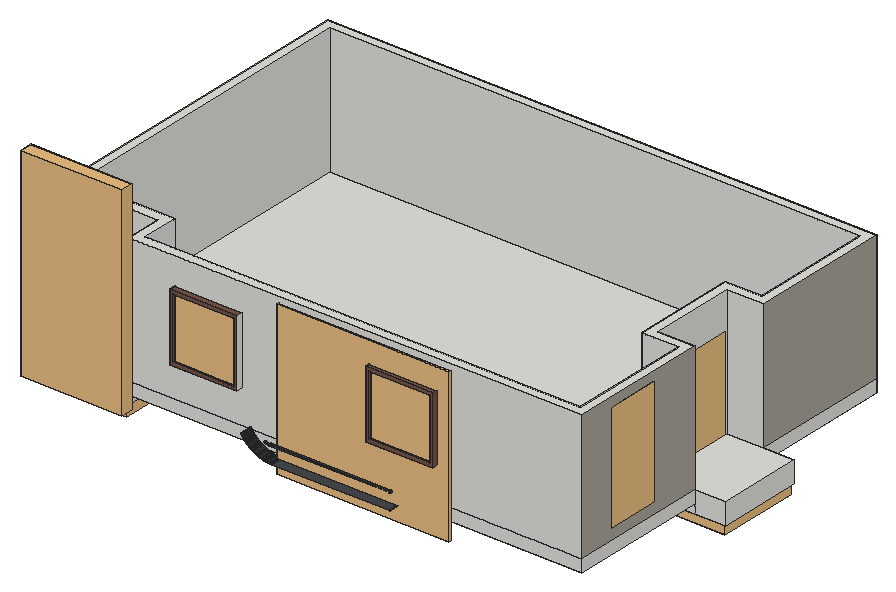
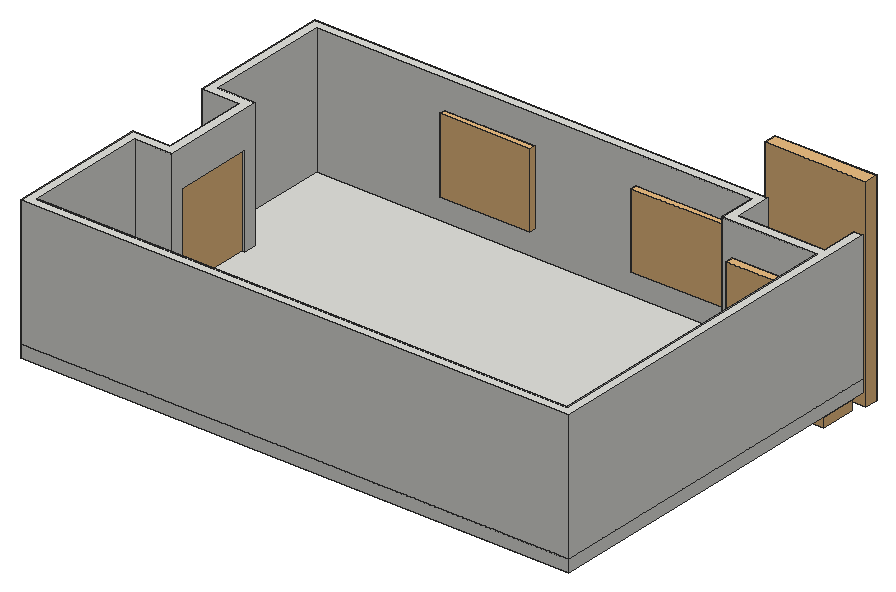
# SketchUp Ruby script. Lengths in inches.
U = 1.inch
M = Sketchup.active_model
def pt(a) = Geom::Point3d.new(a.map { |v| v * U })
def face(e, loops, mat)
  f = e.add_face(loops[0].map { |a| pt(a) })
  loops[1..].each { |l| e.add_face(l.map { |a| pt(a) }).erase! }
  f.material = f.back_material = mat if mat
  f
end
# faces: each face lists its corners as indices into pts; further lists are holes
def faces(e, pts, list, mat = nil) = list.each { |f| face(e, (f[0].is_a?(Array) ? f : [f]).map { |l| l.map { |i| pts[i] } }, mat) }
# xy, xz, yz: faces in a plane at the given z, y or x. An outline is a flat list of corners, or four numbers for a rectangle; further outlines are holes
def ring(l) = l.size == 4 ? [[l[0], l[1]], [l[2], l[1]], [l[2], l[3]], [l[0], l[3]]] : l.each_slice(2).to_a
def flat(e, list, mat, &to3) = list.each { |f| face(e, (f[0].is_a?(Array) ? f : [f]).map { |l| ring(l).map { |u, v| to3.(u, v) } }, mat) }
def xy(e, z, list, mat = nil) = flat(e, list, mat) { |x, y| [x, y, z] }
def xz(e, y, list, mat = nil) = flat(e, list, mat) { |x, z| [x, y, z] }
def yz(e, x, list, mat = nil) = flat(e, list, mat) { |y, z| [x, y, z] }
def lines(e, pts, list) = list.each { |a, b| e.add_line(pt(pts[a]), pt(pts[b])) }
# prism: a flat outline (further loops are holes) pulled along v
def prism(e, loops, v, mat = nil)
  f = face(e, loops, mat); d = Geom::Vector3d.new(v.map { |x| x * U })
  f.pushpull(f.normal.samedirection?(d) ? d.length : -d.length)
end
def box(e, o, s, mat = nil) = prism(e, [[o, [o[0] + s[0], o[1], o[2]], [o[0] + s[0], o[1] + s[1], o[2]], [o[0], o[1] + s[1], o[2]]]], [0, 0, s[2]], mat)
def at(x, y, z, deg = 0) = Geom::Transformation.translation(pt([x, y, z])) * Geom::Transformation.rotation(ORIGIN, Z_AXIS, deg.degrees)
def axes(o, x, y, z) = Geom::Transformation.new([*x, 0, *y, 0, *z, 0, *pt(o).to_a, 1])
def part(name) = M.definitions.add(name)
# library, detail: a bought-in or finely detailed component or shape, given as its bounding box
def library(name, o, s) = part(name).tap { |d| box(d.entities, o, s) }
def detail(e, o, s) = box(e.add_group.entities, o, s)
def put(e, d, t, mat = nil) = e.add_instance(d, t).tap { |i| i.material = mat if mat }
def group(e, t, mat = nil) = e.add_group.tap { |g| g.transformation = t; g.material = mat if mat }.entities
root = M.entities
M.materials.add("1111 AP 9939 Brown seed-N").color = [120, 84, 73]
M.materials.add("1432 AP 8245 TAR ROAD").color = [71, 72, 75]
M.materials.add("Generic").color = [172, 166, 153]
M.materials.add("Outer Light").color = [251, 217, 152]
M.materials.add("[Granite Dark Gray]").color = [69, 68, 68]
M.materials.add("[Wood Cherry Original]").color = [152, 86, 42]
M.materials.add("[Wood Veneer 01]").color = [120, 70, 37]
c1 = library("Group\#45",[0,-2,0],[63,2,36])
c2 = library("Group\#3",[-12,-12.5,-24],[99,12.5,198])
c3 = library("Double-hung window 69 in. x 58 in. triple row with mullions",[0,0,-3.59],[62,58,4.59])
c4 = library("Glass Door",[0,0,0],[72,3.54,96])
c5 = library("RIDEAUX \#16",[0,0,0],[103.86,7.74,93.57])
c6 = library("Curtain",[0,0,0],[121.12,7.86,100.24])
c7 = library("SLIDING+GLASS+DOOR",[0,-0.75,0],[72,5.75,80])
c8 = library("Group\#19",[0,0,0],[0.5,51,105])
c9 = library("Group\#46",[0,-2,0],[168,2,149.16])
c10 = library("Group\#56",[0,0,-17.09],[62,80,17.09])
c11 = library("Group\#32",[0,0,-17.09],[62,80,17.09])
xy(root,428.79,[[278.72,95.37,279,107.37],[279,95.37,393,107.37],[393,95.37,393.24,107.37],[393.24,95.37,393.47,107.37]],"1432 AP 8245 TAR ROAD")
xy(root,428.8,[[278.15,95.37,278.43,107.37]],"1432 AP 8245 TAR ROAD")
xy(root,444.29,[[278.68,95.37,278.84,96.87],[278.84,95.37,279,96.87],[279,95.37,393,96.87],[393,95.37,393.4375,96.87]],"1432 AP 8245 TAR ROAD")
xy(root,444.29,[[278.68,95.37,278.84,96.87],[278.84,95.37,279,96.87],[279,95.37,393,96.87],[393,95.37,393.4375,96.87]],"Outer Light")
xy(root,444.3,[[278.36,95.37,278.52,96.87]],"1432 AP 8245 TAR ROAD")
xy(root,444.3,[[278.36,95.37,278.52,96.87]],"Outer Light")
xy(root,444.31,[[278.03,95.37,278.2,96.87]],"1432 AP 8245 TAR ROAD")
xy(root,444.31,[[278.03,95.37,278.2,96.87]],"Outer Light")
xy(root,445.79,[[278.7,95.37,278.85,96.87],[278.85,95.37,279,96.87],[279,95.37,393,96.87],[393,95.37,393.46,96.87]],"1432 AP 8245 TAR ROAD")
xy(root,445.79,[[278.7,95.37,278.85,96.87],[278.85,95.37,279,96.87],[279,95.37,393,96.87],[393,95.37,393.46,96.87]],"Outer Light")
xy(root,445.8,[[278.4,95.37,278.55,96.87]],"1432 AP 8245 TAR ROAD")
xy(root,445.8,[[278.4,95.37,278.55,96.87]],"Outer Light")
p = [[394.18,107.37,428.75],[394.41,107.37,428.74],[394.41,95.37,428.74],[394.18,95.37,428.75],[394.65,107.37,428.72],[394.65,95.37,428.72],
  [394.88,107.37,428.69],[394.88,95.37,428.69],[276.74,107.37,428.86],[277.02,107.37,428.85],[277.02,95.37,428.85],[276.74,95.37,428.86],
  [277.3,107.37,428.83],[277.3,95.37,428.83],[277.59,107.37,428.82],[277.59,95.37,428.82],[277.87,107.37,428.81],[277.87,95.37,428.81],
  [278.15,107.37,428.8],[278.15,95.37,428.8],[278.43,107.37,428.8],[278.72,107.37,428.79],[278.72,95.37,428.79],[278.43,95.37,428.8],
  [393.47,107.37,428.79],[393.71,107.37,428.78],[393.71,95.37,428.78],[393.47,95.37,428.79],[393.94,107.37,428.77],[393.94,95.37,428.77],
  [275.61,107.37,428.95],[275.89,107.37,428.93],[275.89,95.37,428.93],[275.61,95.37,428.95],[276.18,107.37,428.9],[276.18,95.37,428.9],
  [276.46,107.37,428.88],[276.46,95.37,428.88],[274.49,107.37,429.08],[274.77,107.37,429.04],[274.77,95.37,429.04],[274.49,95.37,429.08],
  [275.05,107.37,429.01],[275.05,95.37,429.01],[275.33,107.37,428.98],[275.33,95.37,428.98],[273.93,107.37,429.15],[274.21,107.37,429.11],
  [274.21,95.37,429.11],[273.93,95.37,429.15],[273.09,107.37,429.28],[273.37,107.37,429.24],[273.37,95.37,429.24],[273.09,95.37,429.28],
  [273.65,107.37,429.19],[273.65,95.37,429.19],[272.53,107.37,429.38],[272.8125,107.37,429.33],[272.8125,95.37,429.33],[272.53,95.37,429.38],
  [271.98,107.37,429.48],[272.25,107.37,429.43],[272.25,95.37,429.43],[271.98,95.37,429.48],[271.42,107.37,429.6],[271.7,107.37,429.54],
  [271.7,95.37,429.54],[271.42,95.37,429.6],[271.15,107.37,429.66],[271.15,95.37,429.66],[270.6,107.37,429.79],[270.87,107.37,429.72],
  [270.87,95.37,429.72],[270.6,95.37,429.79],[270.32,107.37,429.85],[270.32,95.37,429.85],[269.77,107.37,429.99],[270.05,107.37,429.92],
  [270.05,95.37,429.92],[269.77,95.37,429.99],[269.5,107.37,430.07],[269.5,95.37,430.07],[268.96,107.37,430.22],[269.23,107.37,430.14],
  [269.23,95.37,430.14],[268.96,95.37,430.22],[268.69,107.37,430.3],[268.69,95.37,430.3],[268.41,107.37,430.38],[268.41,95.37,430.38],
  [268.14,107.37,430.47],[268.14,95.37,430.47],[267.875,107.37,430.55],[267.875,95.37,430.55],[267.34,107.37,430.73],[267.61,107.37,430.64],
  [267.61,95.37,430.64],[267.34,95.37,430.73],[267.07,107.37,430.83],[267.07,95.37,430.83],[266.81,107.37,430.92],[266.81,95.37,430.92],
  [266.54,107.37,431.02],[266.54,95.37,431.02],[266.27,107.37,431.12],[266.27,95.37,431.12],[266.01,107.37,431.22],[266.01,95.37,431.22],
  [265.75,107.37,431.32],[265.75,95.37,431.32],[265.49,107.37,431.43],[265.49,95.37,431.43],[265.22,107.37,431.53],[265.22,95.37,431.53],
  [264.96,107.37,431.64],[264.96,95.37,431.64],[264.7,107.37,431.75],[264.7,95.37,431.75],[264.44,107.37,431.87],[264.44,95.37,431.87],
  [264.19,107.37,431.98],[264.19,95.37,431.98],[263.93,107.37,432.1],[263.93,95.37,432.1],[263.67,107.37,432.22],[263.67,95.37,432.22],
  [263.42,107.37,432.34],[263.42,95.37,432.34],[263.16,107.37,432.46],[263.16,95.37,432.46],[262.91,107.37,432.59],[262.91,95.37,432.59],
  [262.66,107.37,432.72],[262.66,95.37,432.72],[262.4,107.37,432.85],[262.4,95.37,432.85],[262.15,107.37,432.98],[262.15,95.37,432.98],
  [261.91,107.37,433.11],[261.91,95.37,433.11],[261.66,107.37,433.25],[261.66,95.37,433.25],[261.41,107.37,433.38],[261.41,95.37,433.38],
  [261.16,107.37,433.52],[261.16,95.37,433.52],[260.92,107.37,433.66],[260.92,95.37,433.66],[260.67,107.37,433.81],[260.67,95.37,433.81],
  [260.43,107.37,433.95],[260.43,95.37,433.95],[260.19,107.37,434.1],[260.19,95.37,434.1],[259.95,107.37,434.25],[259.95,95.37,434.25],
  [259.71,107.37,434.4],[259.71,95.37,434.4],[259.47,107.37,434.55],[259.47,95.37,434.55],[259.24,107.37,434.7],[259.24,95.37,434.7],
  [259,107.37,434.86],[259,95.37,434.86],[258.76,107.37,435.02],[258.76,95.37,435.02],[258.53,107.37,435.18],[258.53,95.37,435.18],
  [258.3,107.37,435.34],[258.3,95.37,435.34],[258.07,107.37,435.5],[258.07,95.37,435.5],[257.84,107.37,435.67],[257.84,95.37,435.67],
  [257.61,107.37,435.83],[257.61,95.37,435.83],[257.38,107.37,436],[257.38,95.37,436],[257.16,107.37,436.17],[257.16,95.37,436.17],
  [256.94,107.37,436.35],[256.94,95.37,436.35],[256.71,107.37,436.52],[256.71,95.37,436.52],[256.49,107.37,436.7],[256.49,95.37,436.7],
  [256.27,107.37,436.875],[256.27,95.37,436.875],[256.05,107.37,437.05],[256.05,95.37,437.05],[255.84,107.37,437.23],[255.84,95.37,437.23],
  [255.62,107.37,437.42],[255.62,95.37,437.42],[255.41,107.37,437.6],[255.41,95.37,437.6],[255.19,107.37,437.79],[255.19,95.37,437.79],
  [254.98,107.37,437.98],[254.98,95.37,437.98],[254.77,107.37,438.17],[254.77,95.37,438.17],[254.5625,107.37,438.36],[254.5625,95.37,438.36],
  [254.36,107.37,438.55],[254.36,95.37,438.55],[254.15,107.37,438.74],[254.15,95.37,438.74],[253.95,107.37,438.94],[253.95,95.37,438.94],
  [253.74,107.37,439.14],[253.74,95.37,439.14],[253.54,107.37,439.34],[253.54,95.37,439.34],[253.35,107.37,439.54],[253.35,95.37,439.54],
  [253.15,107.37,439.74],[253.15,95.37,439.74],[252.95,107.37,439.94],[252.95,95.37,439.94],[252.76,107.37,440.15],[252.76,95.37,440.15],
  [252.5625,107.37,440.36],[252.5625,95.37,440.36],[252.375,107.37,440.5625],[252.375,95.37,440.5625],[252.18,107.37,440.77],[252.18,95.37,440.77],
  [252,107.37,440.98],[252,95.37,440.98],[251.81,107.37,441.2],[251.81,95.37,441.2],[251.625,107.37,441.41],[251.625,95.37,441.41],
  [251.44,107.37,441.63],[251.44,95.37,441.63],[251.26,107.37,441.84],[251.26,95.37,441.84],[251.08,107.37,442.0625],[251.08,95.37,442.0625],
  [250.9,107.37,442.28],[250.9,95.37,442.28],[250.73,107.37,442.5],[250.73,95.37,442.5],[250.55,107.37,442.73],[250.55,95.37,442.73],
  [250.38,107.37,442.95],[250.38,95.37,442.95],[250.21,107.37,443.18],[250.21,95.37,443.18],[250.04,107.37,443.4],[250.04,95.37,443.4],
  [249.875,107.37,443.63],[249.875,95.37,443.63],[249.71,107.37,443.86],[249.71,95.37,443.86],[249.55,107.37,444.09],[249.55,95.37,444.09],
  [249.38,107.37,444.32],[249.38,95.37,444.32],[394.32,95.37,444.27],[394.75,95.37,444.25],[394.75,96.87,444.25],[394.32,96.87,444.27],
  [394.32,96.87,444.27],[394.75,96.87,444.25],[394.75,95.37,444.25],[394.32,95.37,444.27],[395.19,95.37,444.22],[395.19,96.87,444.22],
  [249.23,107.37,444.56],[249.23,95.37,444.56],[277.39,95.37,444.36],[277.55,95.37,444.34],[277.55,96.87,444.34],[277.39,96.87,444.36],
  [277.39,96.87,444.36],[277.55,96.87,444.34],[277.55,95.37,444.34],[277.39,95.37,444.36],[277.71,95.37,444.33],[277.71,96.87,444.33],
  [277.71,96.87,444.33],[277.71,95.37,444.33],[277.875,95.37,444.32],[277.875,96.87,444.32],[277.875,96.87,444.32],[277.875,95.37,444.32],
  [278.03,95.37,444.31],[278.03,96.87,444.31],[278.03,96.87,444.31],[278.03,95.37,444.31],[278.2,95.37,444.31],[278.36,95.37,444.3],
  [278.36,96.87,444.3],[278.2,96.87,444.31],[278.2,96.87,444.31],[278.36,96.87,444.3],[278.36,95.37,444.3],[278.2,95.37,444.31],
  [278.52,95.37,444.3],[278.68,95.37,444.29],[278.68,96.87,444.29],[278.52,96.87,444.3],[278.52,96.87,444.3],[278.68,96.87,444.29],
  [278.68,95.37,444.29],[278.52,95.37,444.3],[393.4375,95.37,444.29],[393.875,95.37,444.28],[393.875,96.87,444.28],[393.4375,96.87,444.29],
  [393.4375,96.87,444.29],[393.875,96.87,444.28],[393.875,95.37,444.28],[393.4375,95.37,444.29],[276.43,95.37,444.45],[276.59,95.37,444.43],
  [276.59,96.87,444.43],[276.43,96.87,444.45],[276.43,96.87,444.45],[276.59,96.87,444.43],[276.59,95.37,444.43],[276.43,95.37,444.45],
  [276.75,95.37,444.42],[276.75,96.87,444.42],[276.75,96.87,444.42],[276.75,95.37,444.42],[276.91,95.37,444.4],[276.91,96.87,444.4],
  [276.91,96.87,444.4],[276.91,95.37,444.4],[277.07,95.37,444.38],[277.07,96.87,444.38],[277.07,96.87,444.38],[277.07,95.37,444.38],
  [277.23,95.37,444.37],[277.23,96.87,444.37],[277.23,96.87,444.37],[277.23,95.37,444.37],[275.63,95.37,444.57],[275.79,95.37,444.54],
  [275.79,96.87,444.54],[275.63,96.87,444.57],[275.63,96.87,444.57],[275.79,96.87,444.54],[275.79,95.37,444.54],[275.63,95.37,444.57],
  [275.95,95.37,444.52],[275.95,96.87,444.52],[275.95,96.87,444.52],[275.95,95.37,444.52],[276.11,95.37,444.5],[276.11,96.87,444.5],
  [276.11,96.87,444.5],[276.11,95.37,444.5],[276.27,95.37,444.47],[276.27,96.87,444.47],[276.27,96.87,444.47],[276.27,95.37,444.47],
  [249.07,107.37,444.79],[249.07,95.37,444.79],[275.16,95.37,444.66],[275.32,95.37,444.625],[275.32,96.87,444.625],[275.16,96.87,444.66],
  [275.16,96.87,444.66],[275.32,96.87,444.625],[275.32,95.37,444.625],[275.16,95.37,444.66],[275.48,95.37,444.6],[275.48,96.87,444.6],
  [275.48,96.87,444.6],[275.48,95.37,444.6],[274.69,95.37,444.75],[274.84,95.37,444.72],[274.84,96.87,444.72],[274.69,96.87,444.75],
  [274.69,96.87,444.75],[274.84,96.87,444.72],[274.84,95.37,444.72],[274.69,95.37,444.75],[275,95.37,444.6875],[275,96.87,444.6875],
  [275,96.87,444.6875],[275,95.37,444.6875],[248.91,107.37,445.03],[248.91,95.37,445.03],[274.21,95.37,444.86],[274.37,95.37,444.82],
  [274.37,96.87,444.82],[274.21,96.87,444.86],[274.21,96.87,444.86],[274.37,96.87,444.82],[274.37,95.37,444.82],[274.21,95.37,444.86],
  [274.53,95.37,444.79],[274.53,96.87,444.79],[274.53,96.87,444.79],[274.53,95.37,444.79],[273.75,95.37,444.98],[273.9,95.37,444.9375],
  [273.9,96.87,444.9375],[273.75,96.87,444.98],[273.75,96.87,444.98],[273.9,96.87,444.9375],[273.9,95.37,444.9375],[273.75,95.37,444.98],
  [274.06,95.37,444.9],[274.06,96.87,444.9],[274.06,96.87,444.9],[274.06,95.37,444.9],[248.76,107.37,445.26],[248.76,95.37,445.26],
  [273.44,95.37,445.0625],[273.59,95.37,445.02],[273.59,96.87,445.02],[273.44,96.87,445.0625],[273.44,96.87,445.0625],[273.59,96.87,445.02],
  [273.59,95.37,445.02],[273.44,95.37,445.0625],[273.125,95.37,445.15],[273.28,95.37,445.11],[273.28,96.87,445.11],[273.125,96.87,445.15],
  [273.125,96.87,445.15],[273.28,96.87,445.11],[273.28,95.37,445.11],[273.125,95.37,445.15],[272.67,95.37,445.3],[272.82,95.37,445.25],
  [272.82,96.87,445.25],[272.67,96.87,445.3],[272.67,96.87,445.3],[272.82,96.87,445.25],[272.82,95.37,445.25],[272.67,95.37,445.3],
  [272.97,95.37,445.2],[272.97,96.87,445.2],[272.97,96.87,445.2],[272.97,95.37,445.2],[248.6,107.37,445.5],[248.6,95.37,445.5],
  [272.36,95.37,445.4],[272.51,95.37,445.35],[272.51,96.87,445.35],[272.36,96.87,445.4],[272.36,96.87,445.4],[272.51,96.87,445.35],
  [272.51,95.37,445.35],[272.36,95.37,445.4],[272.21,95.37,445.45],[272.21,96.87,445.45],[272.21,96.87,445.45],[272.21,95.37,445.45],
  [248.45,107.37,445.74],[248.45,95.37,445.74],[271.9,95.37,445.56],[272.06,95.37,445.5],[272.06,96.87,445.5],[271.9,96.87,445.56],
  [271.9,96.87,445.56],[272.06,96.87,445.5],[272.06,95.37,445.5],[271.9,95.37,445.56],[271.6,95.37,445.67],[271.75,95.37,445.62],
  [271.75,96.87,445.62],[271.6,96.87,445.67],[271.6,96.87,445.67],[271.75,96.87,445.62],[271.75,95.37,445.62],[271.6,95.37,445.67],
  [248.3,107.37,445.98],[248.3,95.37,445.98],[271.3,95.37,445.79],[271.45,95.37,445.73],[271.45,96.87,445.73],[271.3,96.87,445.79],
  [271.3,96.87,445.79],[271.45,96.87,445.73],[271.45,95.37,445.73],[271.3,95.37,445.79],[394.83,95.37,445.74],[394.375,95.37,445.77],
  [394.375,96.87,445.77],[394.83,96.87,445.74],[394.83,96.87,445.74],[394.375,96.87,445.77],[394.375,95.37,445.77],[394.83,95.37,445.74],
  [271.15,95.37,445.85],[271.15,96.87,445.85],[271.15,96.87,445.85],[271.15,95.37,445.85],[277.66,95.37,445.84],[277.51,95.37,445.85],
  [277.51,96.87,445.85],[277.66,96.87,445.84],[277.66,96.87,445.84],[277.51,96.87,445.85],[277.51,95.37,445.85],[277.66,95.37,445.84],
  [277.81,95.37,445.83],[277.81,96.87,445.83],[277.81,96.87,445.83],[277.81,95.37,445.83],[277.96,95.37,445.82],[277.96,96.87,445.82],
  [277.96,96.87,445.82],[277.96,95.37,445.82],[278.1,95.37,445.8125],[278.1,96.87,445.8125],[278.1,96.87,445.8125],[278.1,95.37,445.8125],
  [278.25,95.37,445.81],[278.25,96.87,445.81],[278.25,96.87,445.81],[278.25,95.37,445.81],[278.4,95.37,445.8],[278.4,96.87,445.8],
  [278.4,96.87,445.8],[278.4,95.37,445.8],[278.7,95.37,445.79],[278.55,95.37,445.8],[278.55,96.87,445.8],[278.7,96.87,445.79],
  [278.7,96.87,445.79],[278.55,96.87,445.8],[278.55,95.37,445.8],[278.7,95.37,445.79],[393.92,95.37,445.78],[393.46,95.37,445.79],
  [393.46,96.87,445.79],[393.92,96.87,445.78],[393.92,96.87,445.78],[393.46,96.87,445.79],[393.46,95.37,445.79],[393.92,95.37,445.78],
  [271.01,95.37,445.91],[271.01,96.87,445.91],[271.01,96.87,445.91],[271.01,95.37,445.91],[277.0625,95.37,445.89],[276.92,95.37,445.91],
  [276.92,96.87,445.91],[277.0625,96.87,445.89],[277.0625,96.87,445.89],[276.92,96.87,445.91],[276.92,95.37,445.91],[277.0625,95.37,445.89],
  [277.21,95.37,445.875],[277.21,96.87,445.875],[277.21,96.87,445.875],[277.21,95.37,445.875],[277.36,95.37,445.86],[277.36,96.87,445.86],
  [277.36,96.87,445.86],[277.36,95.37,445.86]]
faces(root,p,[[0,1,2,3],[1,4,5,2],[4,6,7,5],[8,9,10,11],[9,12,13,10],[12,14,15,13],[14,16,17,15],[16,18,19,17],
  [20,21,22,23],[24,25,26,27],[25,28,29,26],[28,0,3,29],[30,31,32,33],[31,34,35,32],[34,36,37,35],[36,8,11,37],
  [38,39,40,41],[39,42,43,40],[42,44,45,43],[44,30,33,45],[46,47,48,49],[47,38,41,48],[50,51,52,53],[51,54,55,52],
  [54,46,49,55],[56,57,58,59],[57,50,53,58],[60,61,62,63],[61,56,59,62],[64,65,66,67],[65,60,63,66],[68,64,67,69],
  [70,71,72,73],[71,68,69,72],[74,70,73,75],[76,77,78,79],[77,74,75,78],[80,76,79,81],[82,83,84,85],[83,80,81,84],
  [86,82,85,87],[88,86,87,89],[90,88,89,91],[92,90,91,93],[94,95,96,97],[95,92,93,96],[98,94,97,99],[100,98,99,101],
  [102,100,101,103],[104,102,103,105],[106,104,105,107],[108,106,107,109],[110,108,109,111],[112,110,111,113],[114,112,113,115],[116,114,115,117],
  [118,116,117,119],[120,118,119,121],[122,120,121,123],[124,122,123,125],[126,124,125,127],[128,126,127,129],[130,128,129,131],[132,130,131,133],
  [134,132,133,135],[136,134,135,137],[138,136,137,139],[140,138,139,141],[142,140,141,143],[144,142,143,145],[146,144,145,147],[148,146,147,149],
  [150,148,149,151],[152,150,151,153],[154,152,153,155],[156,154,155,157],[158,156,157,159],[160,158,159,161],[162,160,161,163],[164,162,163,165],
  [166,164,165,167],[168,166,167,169],[170,168,169,171],[172,170,171,173],[174,172,173,175],[176,174,175,177],[178,176,177,179],[180,178,179,181],
  [182,180,181,183],[184,182,183,185],[186,184,185,187],[188,186,187,189],[190,188,189,191],[192,190,191,193],[194,192,193,195],[196,194,195,197],
  [198,196,197,199],[200,198,199,201],[202,200,201,203],[204,202,203,205],[206,204,205,207],[208,206,207,209],[210,208,209,211],[212,210,211,213],
  [214,212,213,215],[216,214,215,217],[218,216,217,219],[220,218,219,221],[222,220,221,223],[224,222,223,225],[226,224,225,227],[228,226,227,229],
  [230,228,229,231],[232,230,231,233],[234,232,233,235],[236,234,235,237],[238,236,237,239],[240,238,239,241],[242,240,241,243],[244,242,243,245],
  [246,244,245,247],[248,246,247,249],[250,248,249,251],[252,250,251,253],[254,252,253,255],[256,254,255,257],[258,256,257,259],[260,261,262,263],
  [261,268,269,262],[270,258,259,271],[272,273,274,275],[273,280,281,274],[280,284,285,281],[284,288,289,285],[292,293,294,295],[300,301,302,303],
  [308,309,310,311],[309,260,263,310],[316,317,318,319],[317,324,325,318],[324,328,329,325],[328,332,333,329],[332,336,337,333],[336,272,275,337],
  [340,341,342,343],[341,348,349,342],[348,352,353,349],[352,356,357,353],[356,316,319,357],[360,270,271,361],[362,363,364,365],[363,370,371,364],
  [370,340,343,371],[374,375,376,377],[375,382,383,376],[382,362,365,383],[386,360,361,387],[388,389,390,391],[389,396,397,390],[396,374,377,397],
  [400,401,402,403],[401,408,409,402],[408,388,391,409],[412,386,387,413],[414,415,416,417],[415,400,403,416],[422,423,424,425],[423,414,417,424],
  [430,431,432,433],[431,438,439,432],[438,422,425,439],[442,412,413,443],[444,445,446,447],[445,430,433,446],[452,444,447,453],[456,442,443,457],
  [458,459,460,461],[459,452,453,460],[466,467,468,469],[467,458,461,468],[474,456,457,475],[476,477,478,479],[477,466,469,478],[484,485,486,487],
  [492,476,479,493],[496,497,498,499],[504,496,499,505],[508,504,505,509],[512,508,509,513],[516,512,513,517],[520,516,517,521],[524,525,526,527],
  [532,533,534,535],[485,532,535,486],[540,492,493,541],[544,545,546,547],[552,544,547,553],[556,552,553,557],[497,556,557,498]],"1432 AP 8245 TAR ROAD")
faces(root,p,[[264,265,266,267],[276,277,278,279],[277,282,283,278],[282,286,287,283],[286,290,291,287],[296,297,298,299],[304,305,306,307],[312,313,314,315],
  [313,264,267,314],[320,321,322,323],[321,326,327,322],[326,330,331,327],[330,334,335,331],[334,338,339,335],[338,276,279,339],[344,345,346,347],
  [345,350,351,346],[350,354,355,351],[354,358,359,355],[358,320,323,359],[366,367,368,369],[367,372,373,368],[372,344,347,373],[378,379,380,381],
  [379,384,385,380],[384,366,369,385],[392,393,394,395],[393,398,399,394],[398,378,381,399],[404,405,406,407],[405,410,411,406],[410,392,395,411],
  [418,419,420,421],[419,404,407,420],[426,427,428,429],[427,418,421,428],[434,435,436,437],[435,440,441,436],[440,426,429,441],[448,449,450,451],
  [449,434,437,450],[454,448,451,455],[462,463,464,465],[463,454,455,464],[470,471,472,473],[471,462,465,472],[480,481,482,483],[481,470,473,482],
  [488,489,490,491],[494,480,483,495],[500,501,502,503],[506,500,503,507],[510,506,507,511],[514,510,511,515],[518,514,515,519],[522,518,519,523],
  [528,529,530,531],[536,537,538,539],[489,536,539,490],[542,494,495,543],[548,549,550,551],[554,548,551,555],[558,554,555,559],[501,558,559,502]],"Outer Light")
put(root,c1,at(51,100.87,443.79),"[Wood Cherry Original]")
put(root,c2,at(45,107.37,443.79),"[Wood Veneer 01]")
g1 = group(root,at(36,101.37,446.79))
xy(g1,-3,[[0,6,9,366],[93,6,537,15],[93,15,102,51],[528,15,528,135,492,135,492,147,501,147,501,144,537,144,537,15],[9,42,24,51],
  [78,42,93,51],[492,225,492,237,528,237,528,357,537,357,537,228,501,228,501,225],[9,357,537,366]])
xy(g1,30,[[138,0,204,6],[330,0,396,6]],"1111 AP 9939 Brown seed-N")
xy(g1,33,[[141,0,201,15],[333,0,393,15]],"1111 AP 9939 Brown seed-N")
xy(g1,81,[[24,42,78,51]])
xy(g1,87,[[492,147,501,225]])
xy(g1,93,[[333,0,393,15]])
xy(g1,93,[[141,0,201,15]],"1111 AP 9939 Brown seed-N")
xy(g1,96,[[138,0,204,6],[330,0,396,6]],"1111 AP 9939 Brown seed-N")
xy(g1,123,[[[0,6,9,6,9,42,93,42,93,6,537,6,537,144,501,144,501,228,537,228,537,366,0,366],[102,15,102,51,9,51,9,357,528,357,528,237,492,237,492,135,528,135,528,15]]])
xz(g1,0,[[[138,30,204,96],[141,33,201,93]],[[330,30,396,96],[333,33,393,93]]],"1111 AP 9939 Brown seed-N")
xz(g1,6,[[0,-3,9,123],[[93,-3,537,123],[330,30,396,96],[138,30,204,96]]])
xz(g1,15,[[[102,-3,528,123],[141,33,201,93],[333,33,393,93]]])
xz(g1,42,[[9,-3,24,-3,24,81,78,81,78,-3,93,-3,93,123,9,123]])
xz(g1,51,[[9,-3,9,123,102,123,102,-3,78,-3,78,81,24,81,24,-3]])
xz(g1,135,[[492,-3,528,123]])
xz(g1,144,[[501,-3,537,123]])
xz(g1,147,[[492,-3,501,87]])
xz(g1,225,[[492,-3,501,87]])
xz(g1,228,[[501,-3,537,123]])
xz(g1,237,[[492,-3,528,123]])
xz(g1,357,[[9,-3,528,123]])
xz(g1,366,[[0,-3,537,123]])
yz(g1,0,[[6,-3,366,123]])
yz(g1,9,[[6,-3,42,123],[51,-3,357,123]])
yz(g1,24,[[42,-3,51,81]])
yz(g1,78,[[42,-3,51,81]])
yz(g1,93,[[6,-3,42,123]])
yz(g1,102,[[15,-3,51,123]])
yz(g1,138,[[0,30,6,96]],"1111 AP 9939 Brown seed-N")
yz(g1,141,[[0,33,15,93]],"1111 AP 9939 Brown seed-N")
yz(g1,201,[[0,33,15,93]],"1111 AP 9939 Brown seed-N")
yz(g1,204,[[0,30,6,96]])
yz(g1,330,[[0,30,6,96]],"1111 AP 9939 Brown seed-N")
yz(g1,333,[[0,33,15,93]],"1111 AP 9939 Brown seed-N")
yz(g1,393,[[0,33,15,93]],"1111 AP 9939 Brown seed-N")
yz(g1,396,[[0,30,6,96]],"1111 AP 9939 Brown seed-N")
yz(g1,492,[[135,-3,135,123,237,123,237,-3,225,-3,225,87,147,87,147,-3]])
yz(g1,501,[[144,-3,147,-3,147,87,225,87,225,-3,228,-3,228,123,144,123]])
yz(g1,528,[[15,-3,135,123],[237,-3,357,123]])
yz(g1,537,[[59.76,9,93,9,93,114,59.76,114,59.53,113.99,59.29,113.99,59.06,113.98,58.82,113.96,58.59,113.94,58.35,113.92,58.12,113.9,57.88,113.875,57.65,113.85,57.42,113.8125,57.18,113.78,56.72,113.7,56.49,113.65,56.26,113.61,56.03,113.56,55.8,113.5,55.57,113.45,55.34,113.39,55.11,113.32,54.89,113.26,54.66,113.19,54.4375,113.12,54.21,113.04,53.99,112.97,53.77,112.89,53.55,112.8,53.33,112.72,52.89,112.54,52.68,112.44,52.46,112.35,52.25,112.25,52.04,112.14,51.83,112.04,51.41,111.82,51.2,111.7,51,111.59,50.6,111.35,50.39,111.22,50.2,111.1,50,110.97,49.8,110.83,49.61,110.7,49.42,110.5625,49.23,110.42,49.04,110.28,48.86,110.14,48.67,109.99,48.49,109.84,48.31,109.6875,48.13,109.53,47.96,109.375,47.78,109.22,47.61,109.06,47.44,108.89,47.27,108.73,47.11,108.56,46.94,108.39,46.78,108.22,46.625,108.04,46.47,107.87,46.3125,107.69,46.16,107.51,46.01,107.33,45.86,107.14,45.72,106.96,45.58,106.77,45.4375,106.58,45.3,106.39,45.17,106.2,45.03,106,44.9,105.8,44.78,105.61,44.65,105.4,44.41,105,44.3,104.8,44.18,104.59,43.96,104.17,43.86,103.96,43.75,103.75,43.65,103.54,43.56,103.32,43.46,103.11,43.28,102.67,43.2,102.45,43.11,102.23,43.03,102.01,42.96,101.79,42.88,101.5625,42.81,101.34,42.74,101.11,42.68,100.89,42.61,100.66,42.55,100.43,42.5,100.2,42.44,99.97,42.39,99.74,42.35,99.51,42.3,99.28,42.22,98.82,42.1875,98.58,42.15,98.35,42.125,98.12,42.1,97.88,42.08,97.65,42.06,97.41,42.04,97.18,42.02,96.94,42.01,96.71,42.01,96.47,42,96.24,42,26.76,42.01,26.53,42.01,26.29,42.02,26.06,42.04,25.82,42.06,25.59,42.08,25.35,42.1,25.12,42.125,24.88,42.15,24.65,42.1875,24.42,42.22,24.18,42.3,23.72,42.35,23.49,42.39,23.26,42.44,23.03,42.5,22.8,42.55,22.57,42.61,22.34,42.68,22.11,42.74,21.89,42.81,21.66,42.88,21.4375,42.96,21.21,43.03,20.99,43.11,20.77,43.2,20.55,43.28,20.33,43.46,19.89,43.56,19.68,43.65,19.46,43.75,19.25,43.86,19.04,43.96,18.83,44.18,18.41,44.3,18.2,44.41,18,44.65,17.6,44.78,17.39,44.9,17.2,45.03,17,45.17,16.8,45.3,16.61,45.4375,16.42,45.58,16.23,45.72,16.04,45.86,15.86,46.01,15.67,46.16,15.49,46.3125,15.31,46.47,15.13,46.625,14.96,46.78,14.78,46.94,14.61,47.11,14.44,47.27,14.27,47.44,14.11,47.61,13.94,47.78,13.78,47.96,13.625,48.13,13.47,48.31,13.3125,48.49,13.16,48.67,13.01,48.86,12.86,49.04,12.72,49.23,12.58,49.42,12.4375,49.61,12.3,49.8,12.17,50,12.03,50.2,11.9,50.39,11.78,50.6,11.65,51,11.41,51.2,11.3,51.41,11.18,51.83,10.96,52.04,10.86,52.25,10.75,52.46,10.65,52.68,10.56,52.89,10.46,53.33,10.28,53.55,10.2,53.77,10.11,53.99,10.03,54.21,9.96,54.4375,9.88,54.66,9.81,54.89,9.74,55.11,9.68,55.34,9.61,55.57,9.55,55.8,9.5,56.03,9.44,56.26,9.39,56.49,9.35,56.72,9.3,57.18,9.22,57.42,9.1875,57.65,9.15,57.88,9.125,58.12,9.1,58.35,9.08,58.59,9.06,58.82,9.04,59.06,9.02,59.29,9.01,59.53,9.01]])
yz(g1,537,[[[6,-3,144,123],[59.76,9,59.53,9.01,59.29,9.01,59.06,9.02,58.82,9.04,58.59,9.06,58.35,9.08,58.12,9.1,57.88,9.125,57.65,9.15,57.42,9.1875,57.18,9.22,56.72,9.3,56.49,9.35,56.26,9.39,56.03,9.44,55.8,9.5,55.57,9.55,55.34,9.61,55.11,9.68,54.89,9.74,54.66,9.81,54.4375,9.88,54.21,9.96,53.99,10.03,53.77,10.11,53.55,10.2,53.33,10.28,52.89,10.46,52.68,10.56,52.46,10.65,52.25,10.75,52.04,10.86,51.83,10.96,51.41,11.18,51.2,11.3,51,11.41,50.6,11.65,50.39,11.78,50.2,11.9,50,12.03,49.8,12.17,49.61,12.3,49.42,12.4375,49.23,12.58,49.04,12.72,48.86,12.86,48.67,13.01,48.49,13.16,48.31,13.3125,48.13,13.47,47.96,13.625,47.78,13.78,47.61,13.94,47.44,14.11,47.27,14.27,47.11,14.44,46.94,14.61,46.78,14.78,46.625,14.96,46.47,15.13,46.3125,15.31,46.16,15.49,46.01,15.67,45.86,15.86,45.72,16.04,45.58,16.23,45.4375,16.42,45.3,16.61,45.17,16.8,45.03,17,44.9,17.2,44.78,17.39,44.65,17.6,44.41,18,44.3,18.2,44.18,18.41,43.96,18.83,43.86,19.04,43.75,19.25,43.65,19.46,43.56,19.68,43.46,19.89,43.28,20.33,43.2,20.55,43.11,20.77,43.03,20.99,42.96,21.21,42.88,21.4375,42.81,21.66,42.74,21.89,42.68,22.11,42.61,22.34,42.55,22.57,42.5,22.8,42.44,23.03,42.39,23.26,42.35,23.49,42.3,23.72,42.22,24.18,42.1875,24.42,42.15,24.65,42.125,24.88,42.1,25.12,42.08,25.35,42.06,25.59,42.04,25.82,42.02,26.06,42.01,26.29,42.01,26.53,42,26.76,42,96.24,42.01,96.47,42.01,96.71,42.02,96.94,42.04,97.18,42.06,97.41,42.08,97.65,42.1,97.88,42.125,98.12,42.15,98.35,42.1875,98.58,42.22,98.82,42.3,99.28,42.35,99.51,42.39,99.74,42.44,99.97,42.5,100.2,42.55,100.43,42.61,100.66,42.68,100.89,42.74,101.11,42.81,101.34,42.88,101.5625,42.96,101.79,43.03,102.01,43.11,102.23,43.2,102.45,43.28,102.67,43.46,103.11,43.56,103.32,43.65,103.54,43.75,103.75,43.86,103.96,43.96,104.17,44.18,104.59,44.3,104.8,44.41,105,44.65,105.4,44.78,105.61,44.9,105.8,45.03,106,45.17,106.2,45.3,106.39,45.4375,106.58,45.58,106.77,45.72,106.96,45.86,107.14,46.01,107.33,46.16,107.51,46.3125,107.69,46.47,107.87,46.625,108.04,46.78,108.22,46.94,108.39,47.11,108.56,47.27,108.73,47.44,108.89,47.61,109.06,47.78,109.22,47.96,109.375,48.13,109.53,48.31,109.6875,48.49,109.84,48.67,109.99,48.86,110.14,49.04,110.28,49.23,110.42,49.42,110.5625,49.61,110.7,49.8,110.83,50,110.97,50.2,111.1,50.39,111.22,50.6,111.35,51,111.59,51.2,111.7,51.41,111.82,51.83,112.04,52.04,112.14,52.25,112.25,52.46,112.35,52.68,112.44,52.89,112.54,53.33,112.72,53.55,112.8,53.77,112.89,53.99,112.97,54.21,113.04,54.4375,113.12,54.66,113.19,54.89,113.26,55.11,113.32,55.34,113.39,55.57,113.45,55.8,113.5,56.03,113.56,56.26,113.61,56.49,113.65,56.72,113.7,57.18,113.78,57.42,113.8125,57.65,113.85,57.88,113.875,58.12,113.9,58.35,113.92,58.59,113.94,58.82,113.96,59.06,113.98,59.29,113.99,59.53,113.99,59.76,114,93,114,93,9]],[228,-3,366,123]],"Generic")
put(g1,c3,axes([201,4.5,33],[-0.96774,0,0],[0,0,1.03448],[0,0.696,0]),"[Granite Dark Gray]")
put(g1,c3,axes([393,4.5,33],[-0.96774,0,0],[0,0,1.03448],[0,0.696,0]),"[Granite Dark Gray]")
put(g1,c4,axes([24,42,-3],[0.75,0,0],[0,0.74,0],[0,0,0.875]))
put(g1,c5,axes([9,51,-3],[0.79912,0,0],[0,1,0],[0,0,1]))
put(g1,c6,axes([126.82,15,21.67],[0.73,0,0],[0,0.73,0],[0,0,0.73]))
put(g1,c6,axes([314.2,15,21.67],[0.73,0,0],[0,0.73,0],[0,0,0.73]))
put(g1,c7,axes([496,225,-3],[0,-1.08333,0],[1,0,0],[0,0,1.125]))
put(g1,c8,at(537,42,9),"[Wood Veneer 01]")
put(g1,c9,at(240,6,-32.16),"Generic")
g2 = group(root,at(45,116.37,431.79))
xy(g2,-9,[[[0,-9,84,27],[2,-7,82,25]],[[492,129,558,213],[494,131,556,211]]])
xy(g2,-3,[[2,-7,82,25]])
xy(g2,-1,[[494,131,556,211]])
xy(g2,0,[[-9,-9,-9,351,528,351,528,213,492,213,492,129,528,129,528,-9,84,-9,84,27,0,27,0,-9]])
xy(g2,12,[[-9,-9,528,-9,528,129,558,129,558,213,528,213,528,351,-9,351]])
xz(g2,-9,[[0,-9,84,-9,84,0,528,0,528,12,-9,12,-9,0,0,0]])
xz(g2,-7,[[2,-9,82,-3]])
xz(g2,25,[[2,-9,82,-3]])
xz(g2,27,[[0,-9,84,0]])
xz(g2,129,[[492,-9,528,0],[528,-9,558,12]])
xz(g2,131,[[494,-9,528,-1],[528,-9,556,-1]])
xz(g2,211,[[494,-9,528,-1],[528,-9,556,-1]])
xz(g2,213,[[492,-9,528,0],[528,-9,558,12]])
xz(g2,351,[[-9,0,528,12]])
yz(g2,-9,[[-9,0,351,12]])
yz(g2,0,[[-9,-9,27,0]])
yz(g2,2,[[-7,-9,25,-3]])
yz(g2,82,[[-7,-9,25,-3]])
yz(g2,84,[[-9,-9,27,0]])
yz(g2,492,[[129,-9,213,0]])
yz(g2,494,[[131,-9,211,-1]])
yz(g2,528,[[-9,0,129,12],[213,0,351,12]])
yz(g2,556,[[131,-9,211,-1]])
yz(g2,558,[[129,-9,213,12]])
put(g2,c10,at(494,131,-1))
put(g2,c11,axes([2,25,-3],[0,-0.54839,0],[1,0,0],[0,0,1]))
